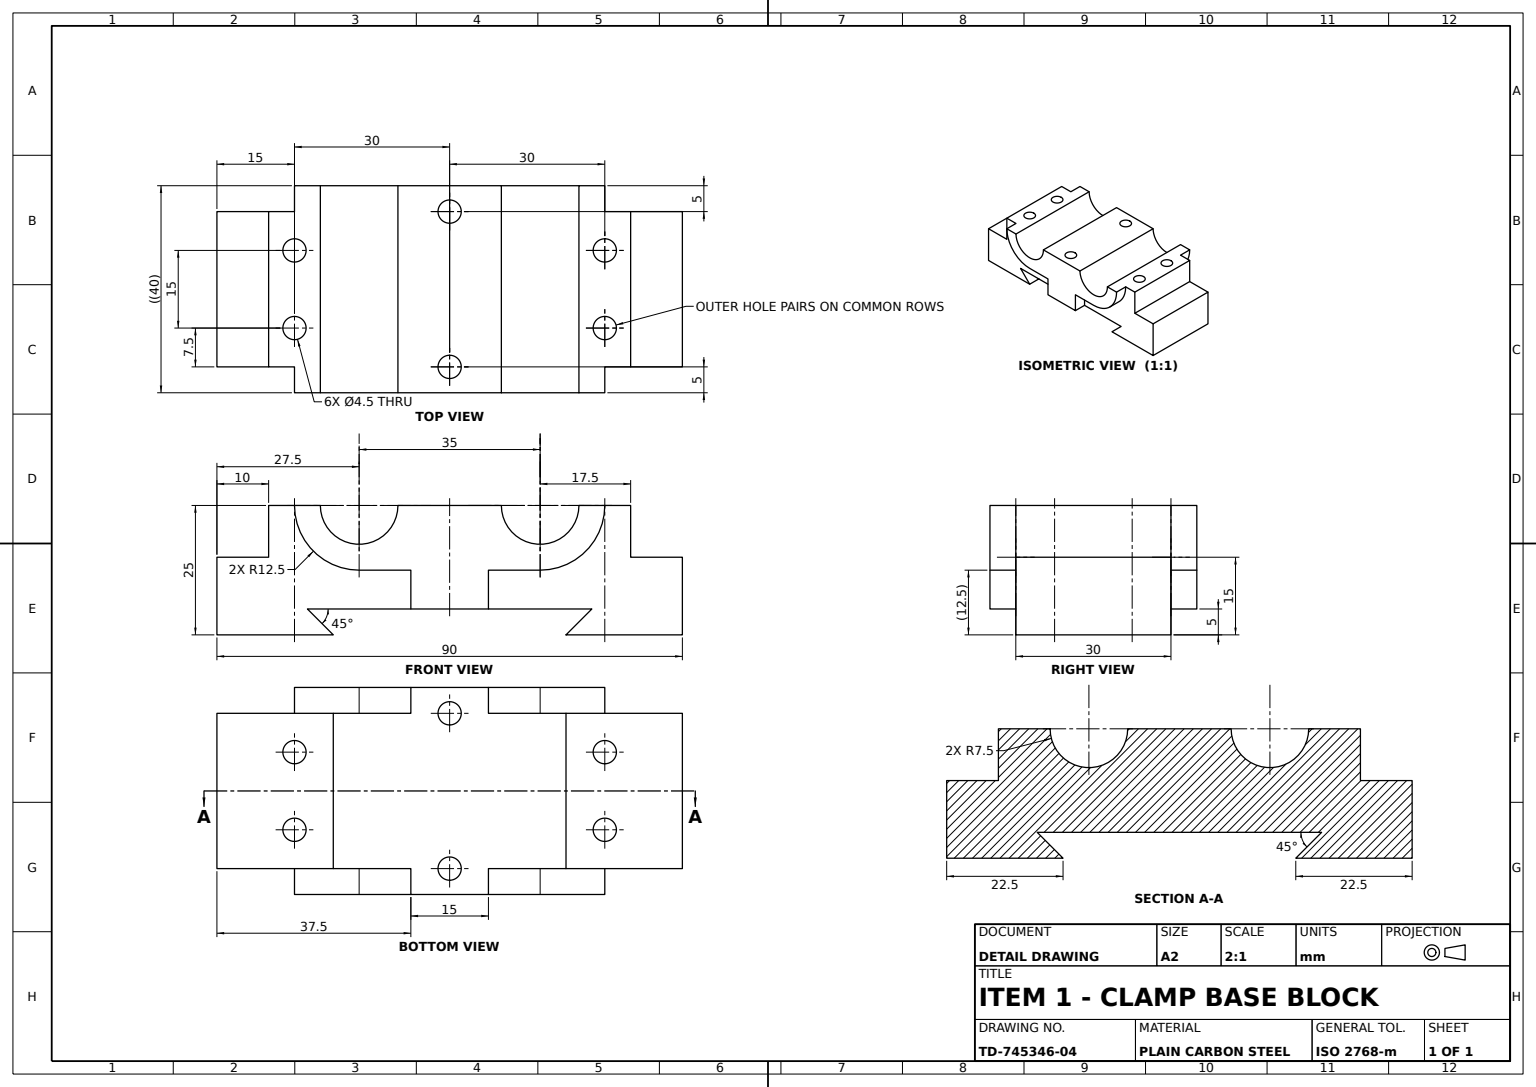
ISO-10303-21;
HEADER;
FILE_DESCRIPTION((''),'2;1');
FILE_NAME('','',(''),(''),'','','');
FILE_SCHEMA(('AUTOMOTIVE_DESIGN'));
ENDSEC;
DATA;
#1=APPLICATION_CONTEXT('');
#2=PRODUCT_CONTEXT('',#1,'mechanical');
#3=PRODUCT('','','',(#2));
#4=PRODUCT_DEFINITION_FORMATION('','',#3);
#5=PRODUCT_DEFINITION_CONTEXT('',#1,'design');
#6=PRODUCT_DEFINITION('','',#4,#5);
#7=PRODUCT_DEFINITION_SHAPE('','',#6);
#8=(LENGTH_UNIT()NAMED_UNIT(*)SI_UNIT(.MILLI.,.METRE.));
#9=(NAMED_UNIT(*)PLANE_ANGLE_UNIT()SI_UNIT($,.RADIAN.));
#10=(NAMED_UNIT(*)SI_UNIT($,.STERADIAN.)SOLID_ANGLE_UNIT());
#11=UNCERTAINTY_MEASURE_WITH_UNIT(LENGTH_MEASURE(1.E-05),#8,'distance_accuracy_value','');
#12=(GEOMETRIC_REPRESENTATION_CONTEXT(3)GLOBAL_UNCERTAINTY_ASSIGNED_CONTEXT((#11))GLOBAL_UNIT_ASSIGNED_CONTEXT((#8,#9,#10))REPRESENTATION_CONTEXT('',''));
#13=CARTESIAN_POINT('',(-25.,18.587361,-20.));
#14=VERTEX_POINT('',#13);
#15=CARTESIAN_POINT('',(-30.,18.587361,-20.));
#16=VERTEX_POINT('',#15);
#17=CARTESIAN_POINT('',(-35.,18.587361,-20.));
#18=DIRECTION('',(-1.,0.,0.));
#19=VECTOR('',#18,1000.);
#20=LINE('',#17,#19);
#21=EDGE_CURVE('',#14,#16,#20,.T.);
#22=ORIENTED_EDGE('',*,*,#21,.F.);
#23=CARTESIAN_POINT('',(-10.,18.587361,-20.));
#24=VERTEX_POINT('',#23);
#25=CARTESIAN_POINT('',(-17.5,18.587361,-20.));
#26=DIRECTION('',(0.,0.,1.));
#27=DIRECTION('',(1.,0.,0.));
#28=AXIS2_PLACEMENT_3D('',#25,#26,#27);
#29=CIRCLE('',#28,7.5);
#30=EDGE_CURVE('',#14,#24,#29,.T.);
#31=ORIENTED_EDGE('',*,*,#30,.T.);
#32=CARTESIAN_POINT('',(10.,18.587361,-20.));
#33=VERTEX_POINT('',#32);
#34=EDGE_CURVE('',#33,#24,#20,.T.);
#35=ORIENTED_EDGE('',*,*,#34,.F.);
#36=CARTESIAN_POINT('',(25.,18.587361,-20.));
#37=VERTEX_POINT('',#36);
#38=CARTESIAN_POINT('',(17.5,18.587361,-20.));
#39=DIRECTION('',(0.,0.,-1.));
#40=AXIS2_PLACEMENT_3D('',#38,#39,#27);
#41=CIRCLE('',#40,7.5);
#42=EDGE_CURVE('',#37,#33,#41,.T.);
#43=ORIENTED_EDGE('',*,*,#42,.F.);
#44=CARTESIAN_POINT('',(30.,18.587361,-20.));
#45=VERTEX_POINT('',#44);
#46=EDGE_CURVE('',#45,#37,#20,.T.);
#47=ORIENTED_EDGE('',*,*,#46,.F.);
#48=CARTESIAN_POINT('',(17.5,6.087361,-20.));
#49=VERTEX_POINT('',#48);
#50=CIRCLE('',#40,12.5);
#51=EDGE_CURVE('',#45,#49,#50,.T.);
#52=ORIENTED_EDGE('',*,*,#51,.T.);
#53=CARTESIAN_POINT('',(7.5,6.087361,-20.));
#54=VERTEX_POINT('',#53);
#55=CARTESIAN_POINT('',(0.,6.087361,-20.));
#56=VECTOR('',#27,1000.);
#57=LINE('',#55,#56);
#58=EDGE_CURVE('',#54,#49,#57,.T.);
#59=ORIENTED_EDGE('',*,*,#58,.F.);
#60=CARTESIAN_POINT('',(7.5,-1.412639,-20.));
#61=VERTEX_POINT('',#60);
#62=CARTESIAN_POINT('',(7.5,0.,-20.));
#63=DIRECTION('',(0.,1.,0.));
#64=VECTOR('',#63,1000.);
#65=LINE('',#62,#64);
#66=EDGE_CURVE('',#61,#54,#65,.T.);
#67=ORIENTED_EDGE('',*,*,#66,.F.);
#68=CARTESIAN_POINT('',(-7.5,-1.412639,-20.));
#69=VERTEX_POINT('',#68);
#70=CARTESIAN_POINT('',(-27.5,-1.412639,-20.));
#71=LINE('',#70,#56);
#72=EDGE_CURVE('',#69,#61,#71,.T.);
#73=ORIENTED_EDGE('',*,*,#72,.F.);
#74=CARTESIAN_POINT('',(-7.5,6.087361,-20.));
#75=VERTEX_POINT('',#74);
#76=CARTESIAN_POINT('',(-7.5,0.,-20.));
#77=LINE('',#76,#64);
#78=EDGE_CURVE('',#69,#75,#77,.T.);
#79=ORIENTED_EDGE('',*,*,#78,.T.);
#80=CARTESIAN_POINT('',(-17.5,6.087361,-20.));
#81=VERTEX_POINT('',#80);
#82=LINE('',#55,#19);
#83=EDGE_CURVE('',#75,#81,#82,.T.);
#84=ORIENTED_EDGE('',*,*,#83,.T.);
#85=CIRCLE('',#28,12.5);
#86=EDGE_CURVE('',#16,#81,#85,.T.);
#87=ORIENTED_EDGE('',*,*,#86,.F.);
#88=EDGE_LOOP('',(#22,#31,#35,#43,#47,#52,#59,#67,#73,#79,#84,#87));
#89=FACE_OUTER_BOUND('',#88,.T.);
#90=CARTESIAN_POINT('',(0.,0.,-20.));
#91=AXIS2_PLACEMENT_3D('',#90,#26,#27);
#92=PLANE('',#91);
#93=ADVANCED_FACE('',(#89),#92,.F.);
#94=CARTESIAN_POINT('',(35.,8.587361,15.));
#95=VERTEX_POINT('',#94);
#96=CARTESIAN_POINT('',(35.,8.587361,-15.));
#97=VERTEX_POINT('',#96);
#98=CARTESIAN_POINT('',(35.,8.587361,20.));
#99=VECTOR('',#39,1000.);
#100=LINE('',#98,#99);
#101=EDGE_CURVE('',#95,#97,#100,.T.);
#102=ORIENTED_EDGE('',*,*,#101,.T.);
#103=CARTESIAN_POINT('',(35.,18.587361,-15.));
#104=VERTEX_POINT('',#103);
#105=DIRECTION('',(0.,-1.,0.));
#106=VECTOR('',#105,1000.);
#107=LINE('',#103,#106);
#108=EDGE_CURVE('',#104,#97,#107,.T.);
#109=ORIENTED_EDGE('',*,*,#108,.F.);
#110=CARTESIAN_POINT('',(35.,18.587361,15.));
#111=VERTEX_POINT('',#110);
#112=CARTESIAN_POINT('',(35.,18.587361,20.));
#113=LINE('',#112,#99);
#114=EDGE_CURVE('',#111,#104,#113,.T.);
#115=ORIENTED_EDGE('',*,*,#114,.F.);
#116=LINE('',#110,#64);
#117=EDGE_CURVE('',#95,#111,#116,.T.);
#118=ORIENTED_EDGE('',*,*,#117,.F.);
#119=EDGE_LOOP('',(#102,#109,#115,#118));
#120=FACE_OUTER_BOUND('',#119,.T.);
#121=AXIS2_PLACEMENT_3D('',#112,#18,#26);
#122=PLANE('',#121);
#123=ADVANCED_FACE('',(#120),#122,.F.);
#124=CARTESIAN_POINT('',(30.,-6.412639,9.75));
#125=VERTEX_POINT('',#124);
#126=CARTESIAN_POINT('',(30.,18.587361,9.75));
#127=VERTEX_POINT('',#126);
#128=CARTESIAN_POINT('',(30.,-21.412639,9.75));
#129=LINE('',#128,#64);
#130=EDGE_CURVE('',#125,#127,#129,.T.);
#131=ORIENTED_EDGE('',*,*,#130,.F.);
#132=CARTESIAN_POINT('',(30.,-6.412639,5.25));
#133=VERTEX_POINT('',#132);
#134=CARTESIAN_POINT('',(30.,-6.412639,7.5));
#135=AXIS2_PLACEMENT_3D('',#134,#63,#18);
#136=CIRCLE('',#135,2.25);
#137=EDGE_CURVE('',#133,#125,#136,.T.);
#138=ORIENTED_EDGE('',*,*,#137,.F.);
#139=CARTESIAN_POINT('',(30.,18.587361,5.25));
#140=VERTEX_POINT('',#139);
#141=CARTESIAN_POINT('',(30.,-21.412639,5.25));
#142=LINE('',#141,#64);
#143=EDGE_CURVE('',#133,#140,#142,.T.);
#144=ORIENTED_EDGE('',*,*,#143,.T.);
#145=CARTESIAN_POINT('',(30.,18.587361,7.5));
#146=AXIS2_PLACEMENT_3D('',#145,#63,#26);
#147=CIRCLE('',#146,2.25);
#148=EDGE_CURVE('',#140,#127,#147,.T.);
#149=ORIENTED_EDGE('',*,*,#148,.T.);
#150=EDGE_LOOP('',(#131,#138,#144,#149));
#151=FACE_OUTER_BOUND('',#150,.T.);
#152=CARTESIAN_POINT('',(30.,-21.412639,7.5));
#153=AXIS2_PLACEMENT_3D('',#152,#63,#26);
#154=CYLINDRICAL_SURFACE('',#153,2.25);
#155=ADVANCED_FACE('',(#151),#154,.F.);
#156=CARTESIAN_POINT('',(-7.5,-1.412639,-15.));
#157=VERTEX_POINT('',#156);
#158=CARTESIAN_POINT('',(-7.5,6.087361,-15.));
#159=VERTEX_POINT('',#158);
#160=CARTESIAN_POINT('',(-7.5,0.,-15.));
#161=LINE('',#160,#64);
#162=EDGE_CURVE('',#157,#159,#161,.T.);
#163=ORIENTED_EDGE('',*,*,#162,.T.);
#164=CARTESIAN_POINT('',(-7.5,6.087361,-125.));
#165=VECTOR('',#26,1000.);
#166=LINE('',#164,#165);
#167=EDGE_CURVE('',#75,#159,#166,.T.);
#168=ORIENTED_EDGE('',*,*,#167,.F.);
#169=ORIENTED_EDGE('',*,*,#78,.F.);
#170=CARTESIAN_POINT('',(-7.5,-1.412639,-125.));
#171=LINE('',#170,#165);
#172=EDGE_CURVE('',#69,#157,#171,.T.);
#173=ORIENTED_EDGE('',*,*,#172,.T.);
#174=EDGE_LOOP('',(#163,#168,#169,#173));
#175=FACE_OUTER_BOUND('',#174,.T.);
#176=CARTESIAN_POINT('',(-7.5,0.,-125.));
#177=AXIS2_PLACEMENT_3D('',#176,#27,#39);
#178=PLANE('',#177);
#179=ADVANCED_FACE('',(#175),#178,.F.);
#180=EDGE_CURVE('',#125,#133,#136,.T.);
#181=ORIENTED_EDGE('',*,*,#180,.F.);
#182=ORIENTED_EDGE('',*,*,#130,.T.);
#183=EDGE_CURVE('',#127,#140,#147,.T.);
#184=ORIENTED_EDGE('',*,*,#183,.T.);
#185=ORIENTED_EDGE('',*,*,#143,.F.);
#186=EDGE_LOOP('',(#181,#182,#184,#185));
#187=FACE_OUTER_BOUND('',#186,.T.);
#188=ADVANCED_FACE('',(#187),#154,.F.);
#189=CARTESIAN_POINT('',(0.,18.587361,-17.25));
#190=VERTEX_POINT('',#189);
#191=CARTESIAN_POINT('',(0.,18.587361,-12.75));
#192=VERTEX_POINT('',#191);
#193=CARTESIAN_POINT('',(0.,18.587361,-15.));
#194=AXIS2_PLACEMENT_3D('',#193,#63,#26);
#195=CIRCLE('',#194,2.25);
#196=EDGE_CURVE('',#190,#192,#195,.T.);
#197=ORIENTED_EDGE('',*,*,#196,.T.);
#198=CARTESIAN_POINT('',(0.,-1.412639,-12.75));
#199=VERTEX_POINT('',#198);
#200=CARTESIAN_POINT('',(0.,-21.412639,-12.75));
#201=LINE('',#200,#64);
#202=EDGE_CURVE('',#199,#192,#201,.T.);
#203=ORIENTED_EDGE('',*,*,#202,.F.);
#204=CARTESIAN_POINT('',(0.,-1.412639,-17.25));
#205=VERTEX_POINT('',#204);
#206=CARTESIAN_POINT('',(0.,-1.412639,-15.));
#207=AXIS2_PLACEMENT_3D('',#206,#63,#18);
#208=CIRCLE('',#207,2.25);
#209=EDGE_CURVE('',#205,#199,#208,.T.);
#210=ORIENTED_EDGE('',*,*,#209,.F.);
#211=CARTESIAN_POINT('',(0.,-21.412639,-17.25));
#212=LINE('',#211,#64);
#213=EDGE_CURVE('',#205,#190,#212,.T.);
#214=ORIENTED_EDGE('',*,*,#213,.T.);
#215=EDGE_LOOP('',(#197,#203,#210,#214));
#216=FACE_OUTER_BOUND('',#215,.T.);
#217=CARTESIAN_POINT('',(0.,-21.412639,-15.));
#218=AXIS2_PLACEMENT_3D('',#217,#63,#26);
#219=CYLINDRICAL_SURFACE('',#218,2.25);
#220=ADVANCED_FACE('',(#216),#219,.F.);
#221=CARTESIAN_POINT('',(-30.,-6.412639,5.25));
#222=VERTEX_POINT('',#221);
#223=CARTESIAN_POINT('',(-30.,18.587361,5.25));
#224=VERTEX_POINT('',#223);
#225=CARTESIAN_POINT('',(-30.,-21.412639,5.25));
#226=LINE('',#225,#64);
#227=EDGE_CURVE('',#222,#224,#226,.T.);
#228=ORIENTED_EDGE('',*,*,#227,.T.);
#229=CARTESIAN_POINT('',(-30.,18.587361,9.75));
#230=VERTEX_POINT('',#229);
#231=CARTESIAN_POINT('',(-30.,18.587361,7.5));
#232=AXIS2_PLACEMENT_3D('',#231,#63,#39);
#233=CIRCLE('',#232,2.25);
#234=EDGE_CURVE('',#224,#230,#233,.T.);
#235=ORIENTED_EDGE('',*,*,#234,.T.);
#236=CARTESIAN_POINT('',(-30.,-6.412639,9.75));
#237=VERTEX_POINT('',#236);
#238=CARTESIAN_POINT('',(-30.,-21.412639,9.75));
#239=LINE('',#238,#64);
#240=EDGE_CURVE('',#237,#230,#239,.T.);
#241=ORIENTED_EDGE('',*,*,#240,.F.);
#242=CARTESIAN_POINT('',(-30.,-6.412639,7.5));
#243=AXIS2_PLACEMENT_3D('',#242,#63,#18);
#244=CIRCLE('',#243,2.25);
#245=EDGE_CURVE('',#222,#237,#244,.T.);
#246=ORIENTED_EDGE('',*,*,#245,.F.);
#247=EDGE_LOOP('',(#228,#235,#241,#246));
#248=FACE_OUTER_BOUND('',#247,.T.);
#249=CARTESIAN_POINT('',(-30.,-21.412639,7.5));
#250=AXIS2_PLACEMENT_3D('',#249,#63,#26);
#251=CYLINDRICAL_SURFACE('',#250,2.25);
#252=ADVANCED_FACE('',(#248),#251,.F.);
#253=CARTESIAN_POINT('',(-30.,18.587361,-9.75));
#254=VERTEX_POINT('',#253);
#255=CARTESIAN_POINT('',(-30.,18.587361,-5.25));
#256=VERTEX_POINT('',#255);
#257=CARTESIAN_POINT('',(-30.,18.587361,-7.5));
#258=AXIS2_PLACEMENT_3D('',#257,#63,#26);
#259=CIRCLE('',#258,2.25);
#260=EDGE_CURVE('',#254,#256,#259,.T.);
#261=ORIENTED_EDGE('',*,*,#260,.T.);
#262=CARTESIAN_POINT('',(-30.,-6.412639,-5.25));
#263=VERTEX_POINT('',#262);
#264=CARTESIAN_POINT('',(-30.,-21.412639,-5.25));
#265=LINE('',#264,#64);
#266=EDGE_CURVE('',#263,#256,#265,.T.);
#267=ORIENTED_EDGE('',*,*,#266,.F.);
#268=CARTESIAN_POINT('',(-30.,-6.412639,-9.75));
#269=VERTEX_POINT('',#268);
#270=CARTESIAN_POINT('',(-30.,-6.412639,-7.5));
#271=AXIS2_PLACEMENT_3D('',#270,#63,#18);
#272=CIRCLE('',#271,2.25);
#273=EDGE_CURVE('',#269,#263,#272,.T.);
#274=ORIENTED_EDGE('',*,*,#273,.F.);
#275=CARTESIAN_POINT('',(-30.,-21.412639,-9.75));
#276=LINE('',#275,#64);
#277=EDGE_CURVE('',#269,#254,#276,.T.);
#278=ORIENTED_EDGE('',*,*,#277,.T.);
#279=EDGE_LOOP('',(#261,#267,#274,#278));
#280=FACE_OUTER_BOUND('',#279,.T.);
#281=CARTESIAN_POINT('',(-30.,-21.412639,-7.5));
#282=AXIS2_PLACEMENT_3D('',#281,#63,#26);
#283=CYLINDRICAL_SURFACE('',#282,2.25);
#284=ADVANCED_FACE('',(#280),#283,.F.);
#285=CARTESIAN_POINT('',(-30.,18.587361,-15.));
#286=VERTEX_POINT('',#285);
#287=CARTESIAN_POINT('',(-35.,18.587361,-15.));
#288=VERTEX_POINT('',#287);
#289=LINE('',#285,#19);
#290=EDGE_CURVE('',#286,#288,#289,.T.);
#291=ORIENTED_EDGE('',*,*,#290,.F.);
#292=CARTESIAN_POINT('',(-17.5,6.087361,-15.));
#293=VERTEX_POINT('',#292);
#294=CARTESIAN_POINT('',(-17.5,18.587361,-15.));
#295=AXIS2_PLACEMENT_3D('',#294,#26,#27);
#296=CIRCLE('',#295,12.5);
#297=EDGE_CURVE('',#286,#293,#296,.T.);
#298=ORIENTED_EDGE('',*,*,#297,.T.);
#299=CARTESIAN_POINT('',(0.,6.087361,-15.));
#300=LINE('',#299,#19);
#301=EDGE_CURVE('',#159,#293,#300,.T.);
#302=ORIENTED_EDGE('',*,*,#301,.F.);
#303=ORIENTED_EDGE('',*,*,#162,.F.);
#304=CARTESIAN_POINT('',(-27.5,-1.412639,-15.));
#305=VERTEX_POINT('',#304);
#306=LINE('',#206,#19);
#307=EDGE_CURVE('',#157,#305,#306,.T.);
#308=ORIENTED_EDGE('',*,*,#307,.T.);
#309=CARTESIAN_POINT('',(-22.5,-6.412639,-15.));
#310=VERTEX_POINT('',#309);
#311=CARTESIAN_POINT('',(-14.45632,-14.45632,-15.));
#312=DIRECTION('',(0.707106781,-0.707106781,0.));
#313=VECTOR('',#312,1000.);
#314=LINE('',#311,#313);
#315=EDGE_CURVE('',#305,#310,#314,.T.);
#316=ORIENTED_EDGE('',*,*,#315,.T.);
#317=CARTESIAN_POINT('',(-45.,-6.412639,-15.));
#318=VERTEX_POINT('',#317);
#319=LINE('',#317,#19);
#320=EDGE_CURVE('',#310,#318,#319,.T.);
#321=ORIENTED_EDGE('',*,*,#320,.T.);
#322=CARTESIAN_POINT('',(-45.,8.587361,-15.));
#323=VERTEX_POINT('',#322);
#324=CARTESIAN_POINT('',(-45.,-21.412639,-15.));
#325=LINE('',#324,#64);
#326=EDGE_CURVE('',#318,#323,#325,.T.);
#327=ORIENTED_EDGE('',*,*,#326,.T.);
#328=CARTESIAN_POINT('',(-35.,8.587361,-15.));
#329=VERTEX_POINT('',#328);
#330=LINE('',#328,#56);
#331=EDGE_CURVE('',#323,#329,#330,.T.);
#332=ORIENTED_EDGE('',*,*,#331,.T.);
#333=LINE('',#287,#64);
#334=EDGE_CURVE('',#329,#288,#333,.T.);
#335=ORIENTED_EDGE('',*,*,#334,.T.);
#336=EDGE_LOOP('',(#291,#298,#302,#303,#308,#316,#321,#327,#332,#335));
#337=FACE_OUTER_BOUND('',#336,.T.);
#338=CARTESIAN_POINT('',(-30.,-21.412639,-15.));
#339=AXIS2_PLACEMENT_3D('',#338,#39,#18);
#340=PLANE('',#339);
#341=ADVANCED_FACE('',(#337),#340,.T.);
#342=ORIENTED_EDGE('',*,*,#326,.F.);
#343=CARTESIAN_POINT('',(-45.,-6.412639,15.));
#344=VERTEX_POINT('',#343);
#345=CARTESIAN_POINT('',(-45.,-6.412639,20.));
#346=LINE('',#345,#99);
#347=EDGE_CURVE('',#344,#318,#346,.T.);
#348=ORIENTED_EDGE('',*,*,#347,.F.);
#349=CARTESIAN_POINT('',(-45.,8.587361,15.));
#350=VERTEX_POINT('',#349);
#351=CARTESIAN_POINT('',(-45.,-21.412639,15.));
#352=LINE('',#351,#64);
#353=EDGE_CURVE('',#344,#350,#352,.T.);
#354=ORIENTED_EDGE('',*,*,#353,.T.);
#355=CARTESIAN_POINT('',(-45.,8.587361,20.));
#356=LINE('',#355,#99);
#357=EDGE_CURVE('',#350,#323,#356,.T.);
#358=ORIENTED_EDGE('',*,*,#357,.T.);
#359=EDGE_LOOP('',(#342,#348,#354,#358));
#360=FACE_OUTER_BOUND('',#359,.T.);
#361=AXIS2_PLACEMENT_3D('',#355,#27,#39);
#362=PLANE('',#361);
#363=ADVANCED_FACE('',(#360),#362,.F.);
#364=CARTESIAN_POINT('',(30.,18.587361,15.));
#365=VERTEX_POINT('',#364);
#366=CARTESIAN_POINT('',(17.5,6.087361,15.));
#367=VERTEX_POINT('',#366);
#368=CARTESIAN_POINT('',(17.5,18.587361,15.));
#369=AXIS2_PLACEMENT_3D('',#368,#39,#18);
#370=CIRCLE('',#369,12.5);
#371=EDGE_CURVE('',#365,#367,#370,.T.);
#372=ORIENTED_EDGE('',*,*,#371,.T.);
#373=CARTESIAN_POINT('',(7.5,6.087361,15.));
#374=VERTEX_POINT('',#373);
#375=CARTESIAN_POINT('',(0.,6.087361,15.));
#376=LINE('',#375,#56);
#377=EDGE_CURVE('',#374,#367,#376,.T.);
#378=ORIENTED_EDGE('',*,*,#377,.F.);
#379=CARTESIAN_POINT('',(7.5,-1.412639,15.));
#380=VERTEX_POINT('',#379);
#381=CARTESIAN_POINT('',(7.5,0.,15.));
#382=LINE('',#381,#64);
#383=EDGE_CURVE('',#380,#374,#382,.T.);
#384=ORIENTED_EDGE('',*,*,#383,.F.);
#385=CARTESIAN_POINT('',(27.5,-1.412639,15.));
#386=VERTEX_POINT('',#385);
#387=CARTESIAN_POINT('',(0.,-1.412639,15.));
#388=LINE('',#387,#56);
#389=EDGE_CURVE('',#380,#386,#388,.T.);
#390=ORIENTED_EDGE('',*,*,#389,.T.);
#391=CARTESIAN_POINT('',(22.5,-6.412639,15.));
#392=VERTEX_POINT('',#391);
#393=CARTESIAN_POINT('',(14.45632,-14.45632,15.));
#394=DIRECTION('',(-0.707106781,-0.707106781,0.));
#395=VECTOR('',#394,1000.);
#396=LINE('',#393,#395);
#397=EDGE_CURVE('',#386,#392,#396,.T.);
#398=ORIENTED_EDGE('',*,*,#397,.T.);
#399=CARTESIAN_POINT('',(45.,-6.412639,15.));
#400=VERTEX_POINT('',#399);
#401=LINE('',#399,#56);
#402=EDGE_CURVE('',#392,#400,#401,.T.);
#403=ORIENTED_EDGE('',*,*,#402,.T.);
#404=CARTESIAN_POINT('',(45.,8.587361,15.));
#405=VERTEX_POINT('',#404);
#406=CARTESIAN_POINT('',(45.,-21.412639,15.));
#407=LINE('',#406,#64);
#408=EDGE_CURVE('',#400,#405,#407,.T.);
#409=ORIENTED_EDGE('',*,*,#408,.T.);
#410=LINE('',#94,#19);
#411=EDGE_CURVE('',#405,#95,#410,.T.);
#412=ORIENTED_EDGE('',*,*,#411,.T.);
#413=ORIENTED_EDGE('',*,*,#117,.T.);
#414=CARTESIAN_POINT('',(45.,18.587361,15.));
#415=LINE('',#414,#56);
#416=EDGE_CURVE('',#365,#111,#415,.T.);
#417=ORIENTED_EDGE('',*,*,#416,.F.);
#418=EDGE_LOOP('',(#372,#378,#384,#390,#398,#403,#409,#412,#413,#417));
#419=FACE_OUTER_BOUND('',#418,.T.);
#420=AXIS2_PLACEMENT_3D('',#406,#26,#27);
#421=PLANE('',#420);
#422=ADVANCED_FACE('',(#419),#421,.T.);
#423=ORIENTED_EDGE('',*,*,#213,.F.);
#424=EDGE_CURVE('',#199,#205,#208,.T.);
#425=ORIENTED_EDGE('',*,*,#424,.F.);
#426=ORIENTED_EDGE('',*,*,#202,.T.);
#427=EDGE_CURVE('',#192,#190,#195,.T.);
#428=ORIENTED_EDGE('',*,*,#427,.T.);
#429=EDGE_LOOP('',(#423,#425,#426,#428));
#430=FACE_OUTER_BOUND('',#429,.T.);
#431=ADVANCED_FACE('',(#430),#219,.F.);
#432=CARTESIAN_POINT('',(-17.5,6.087361,-125.));
#433=LINE('',#432,#165);
#434=EDGE_CURVE('',#81,#293,#433,.T.);
#435=ORIENTED_EDGE('',*,*,#434,.F.);
#436=ORIENTED_EDGE('',*,*,#83,.F.);
#437=ORIENTED_EDGE('',*,*,#167,.T.);
#438=ORIENTED_EDGE('',*,*,#301,.T.);
#439=EDGE_LOOP('',(#435,#436,#437,#438));
#440=FACE_OUTER_BOUND('',#439,.T.);
#441=CARTESIAN_POINT('',(0.,6.087361,-125.));
#442=AXIS2_PLACEMENT_3D('',#441,#63,#18);
#443=PLANE('',#442);
#444=ADVANCED_FACE('',(#440),#443,.F.);
#445=ORIENTED_EDGE('',*,*,#34,.T.);
#446=CARTESIAN_POINT('',(-10.,18.587361,20.));
#447=VERTEX_POINT('',#446);
#448=CARTESIAN_POINT('',(-10.,18.587361,-40.));
#449=LINE('',#448,#165);
#450=EDGE_CURVE('',#24,#447,#449,.T.);
#451=ORIENTED_EDGE('',*,*,#450,.T.);
#452=CARTESIAN_POINT('',(10.,18.587361,20.));
#453=VERTEX_POINT('',#452);
#454=LINE('',#112,#19);
#455=EDGE_CURVE('',#453,#447,#454,.T.);
#456=ORIENTED_EDGE('',*,*,#455,.F.);
#457=CARTESIAN_POINT('',(10.,18.587361,-40.));
#458=LINE('',#457,#165);
#459=EDGE_CURVE('',#33,#453,#458,.T.);
#460=ORIENTED_EDGE('',*,*,#459,.F.);
#461=EDGE_LOOP('',(#445,#451,#456,#460));
#462=FACE_OUTER_BOUND('',#461,.T.);
#463=ORIENTED_EDGE('',*,*,#427,.F.);
#464=ORIENTED_EDGE('',*,*,#196,.F.);
#465=EDGE_LOOP('',(#463,#464));
#466=FACE_BOUND('',#465,.T.);
#467=CARTESIAN_POINT('',(0.,18.587361,17.25));
#468=VERTEX_POINT('',#467);
#469=CARTESIAN_POINT('',(0.,18.587361,12.75));
#470=VERTEX_POINT('',#469);
#471=CARTESIAN_POINT('',(0.,18.587361,15.));
#472=AXIS2_PLACEMENT_3D('',#471,#63,#39);
#473=CIRCLE('',#472,2.25);
#474=EDGE_CURVE('',#468,#470,#473,.T.);
#475=ORIENTED_EDGE('',*,*,#474,.F.);
#476=EDGE_CURVE('',#470,#468,#473,.T.);
#477=ORIENTED_EDGE('',*,*,#476,.F.);
#478=EDGE_LOOP('',(#475,#477));
#479=FACE_BOUND('',#478,.T.);
#480=CARTESIAN_POINT('',(-35.,18.587361,20.));
#481=AXIS2_PLACEMENT_3D('',#480,#105,#39);
#482=PLANE('',#481);
#483=ADVANCED_FACE('',(#462,#466,#479),#482,.F.);
#484=CARTESIAN_POINT('',(-7.5,-1.412639,15.));
#485=VERTEX_POINT('',#484);
#486=CARTESIAN_POINT('',(-7.5,-1.412639,20.));
#487=VERTEX_POINT('',#486);
#488=LINE('',#486,#165);
#489=EDGE_CURVE('',#485,#487,#488,.T.);
#490=ORIENTED_EDGE('',*,*,#489,.T.);
#491=CARTESIAN_POINT('',(-7.5,6.087361,20.));
#492=VERTEX_POINT('',#491);
#493=CARTESIAN_POINT('',(-7.5,0.,20.));
#494=LINE('',#493,#106);
#495=EDGE_CURVE('',#492,#487,#494,.T.);
#496=ORIENTED_EDGE('',*,*,#495,.F.);
#497=CARTESIAN_POINT('',(-7.5,6.087361,15.));
#498=VERTEX_POINT('',#497);
#499=CARTESIAN_POINT('',(-7.5,6.087361,125.));
#500=LINE('',#499,#99);
#501=EDGE_CURVE('',#492,#498,#500,.T.);
#502=ORIENTED_EDGE('',*,*,#501,.T.);
#503=CARTESIAN_POINT('',(-7.5,0.,15.));
#504=LINE('',#503,#64);
#505=EDGE_CURVE('',#485,#498,#504,.T.);
#506=ORIENTED_EDGE('',*,*,#505,.F.);
#507=EDGE_LOOP('',(#490,#496,#502,#506));
#508=FACE_OUTER_BOUND('',#507,.T.);
#509=CARTESIAN_POINT('',(-7.5,0.,125.));
#510=AXIS2_PLACEMENT_3D('',#509,#18,#26);
#511=PLANE('',#510);
#512=ADVANCED_FACE('',(#508),#511,.T.);
#513=CARTESIAN_POINT('',(0.,-1.412639,17.25));
#514=VERTEX_POINT('',#513);
#515=CARTESIAN_POINT('',(0.,-1.412639,12.75));
#516=VERTEX_POINT('',#515);
#517=AXIS2_PLACEMENT_3D('',#387,#63,#18);
#518=CIRCLE('',#517,2.25);
#519=EDGE_CURVE('',#514,#516,#518,.T.);
#520=ORIENTED_EDGE('',*,*,#519,.F.);
#521=CARTESIAN_POINT('',(0.,-21.412639,17.25));
#522=LINE('',#521,#64);
#523=EDGE_CURVE('',#514,#468,#522,.T.);
#524=ORIENTED_EDGE('',*,*,#523,.T.);
#525=ORIENTED_EDGE('',*,*,#474,.T.);
#526=CARTESIAN_POINT('',(0.,-21.412639,12.75));
#527=LINE('',#526,#64);
#528=EDGE_CURVE('',#516,#470,#527,.T.);
#529=ORIENTED_EDGE('',*,*,#528,.F.);
#530=EDGE_LOOP('',(#520,#524,#525,#529));
#531=FACE_OUTER_BOUND('',#530,.T.);
#532=CARTESIAN_POINT('',(0.,-21.412639,15.));
#533=AXIS2_PLACEMENT_3D('',#532,#63,#26);
#534=CYLINDRICAL_SURFACE('',#533,2.25);
#535=ADVANCED_FACE('',(#531),#534,.F.);
#536=ORIENTED_EDGE('',*,*,#408,.F.);
#537=CARTESIAN_POINT('',(45.,-6.412639,-15.));
#538=VERTEX_POINT('',#537);
#539=CARTESIAN_POINT('',(45.,-6.412639,20.));
#540=LINE('',#539,#99);
#541=EDGE_CURVE('',#400,#538,#540,.T.);
#542=ORIENTED_EDGE('',*,*,#541,.T.);
#543=CARTESIAN_POINT('',(45.,8.587361,-15.));
#544=VERTEX_POINT('',#543);
#545=CARTESIAN_POINT('',(45.,-21.412639,-15.));
#546=LINE('',#545,#64);
#547=EDGE_CURVE('',#538,#544,#546,.T.);
#548=ORIENTED_EDGE('',*,*,#547,.T.);
#549=CARTESIAN_POINT('',(45.,8.587361,20.));
#550=LINE('',#549,#99);
#551=EDGE_CURVE('',#405,#544,#550,.T.);
#552=ORIENTED_EDGE('',*,*,#551,.F.);
#553=EDGE_LOOP('',(#536,#542,#548,#552));
#554=FACE_OUTER_BOUND('',#553,.T.);
#555=AXIS2_PLACEMENT_3D('',#549,#18,#26);
#556=PLANE('',#555);
#557=ADVANCED_FACE('',(#554),#556,.F.);
#558=ORIENTED_EDGE('',*,*,#501,.F.);
#559=CARTESIAN_POINT('',(-17.5,6.087361,20.));
#560=VERTEX_POINT('',#559);
#561=CARTESIAN_POINT('',(0.,6.087361,20.));
#562=LINE('',#561,#56);
#563=EDGE_CURVE('',#560,#492,#562,.T.);
#564=ORIENTED_EDGE('',*,*,#563,.F.);
#565=CARTESIAN_POINT('',(-17.5,6.087361,15.));
#566=VERTEX_POINT('',#565);
#567=CARTESIAN_POINT('',(-17.5,6.087361,125.));
#568=LINE('',#567,#99);
#569=EDGE_CURVE('',#560,#566,#568,.T.);
#570=ORIENTED_EDGE('',*,*,#569,.T.);
#571=LINE('',#375,#19);
#572=EDGE_CURVE('',#498,#566,#571,.T.);
#573=ORIENTED_EDGE('',*,*,#572,.F.);
#574=EDGE_LOOP('',(#558,#564,#570,#573));
#575=FACE_OUTER_BOUND('',#574,.T.);
#576=CARTESIAN_POINT('',(0.,6.087361,125.));
#577=AXIS2_PLACEMENT_3D('',#576,#105,#27);
#578=PLANE('',#577);
#579=ADVANCED_FACE('',(#575),#578,.T.);
#580=CARTESIAN_POINT('',(22.5,-6.412639,-15.));
#581=VERTEX_POINT('',#580);
#582=LINE('',#537,#19);
#583=EDGE_CURVE('',#538,#581,#582,.T.);
#584=ORIENTED_EDGE('',*,*,#583,.T.);
#585=CARTESIAN_POINT('',(27.5,-1.412639,-15.));
#586=VERTEX_POINT('',#585);
#587=CARTESIAN_POINT('',(14.45632,-14.45632,-15.));
#588=LINE('',#587,#395);
#589=EDGE_CURVE('',#586,#581,#588,.T.);
#590=ORIENTED_EDGE('',*,*,#589,.F.);
#591=CARTESIAN_POINT('',(7.5,-1.412639,-15.));
#592=VERTEX_POINT('',#591);
#593=LINE('',#206,#56);
#594=EDGE_CURVE('',#592,#586,#593,.T.);
#595=ORIENTED_EDGE('',*,*,#594,.F.);
#596=CARTESIAN_POINT('',(7.5,6.087361,-15.));
#597=VERTEX_POINT('',#596);
#598=CARTESIAN_POINT('',(7.5,0.,-15.));
#599=LINE('',#598,#64);
#600=EDGE_CURVE('',#592,#597,#599,.T.);
#601=ORIENTED_EDGE('',*,*,#600,.T.);
#602=CARTESIAN_POINT('',(17.5,6.087361,-15.));
#603=VERTEX_POINT('',#602);
#604=LINE('',#299,#56);
#605=EDGE_CURVE('',#597,#603,#604,.T.);
#606=ORIENTED_EDGE('',*,*,#605,.T.);
#607=CARTESIAN_POINT('',(30.,18.587361,-15.));
#608=VERTEX_POINT('',#607);
#609=CARTESIAN_POINT('',(17.5,18.587361,-15.));
#610=AXIS2_PLACEMENT_3D('',#609,#39,#18);
#611=CIRCLE('',#610,12.5);
#612=EDGE_CURVE('',#608,#603,#611,.T.);
#613=ORIENTED_EDGE('',*,*,#612,.F.);
#614=LINE('',#607,#19);
#615=EDGE_CURVE('',#104,#608,#614,.T.);
#616=ORIENTED_EDGE('',*,*,#615,.F.);
#617=ORIENTED_EDGE('',*,*,#108,.T.);
#618=LINE('',#96,#56);
#619=EDGE_CURVE('',#97,#544,#618,.T.);
#620=ORIENTED_EDGE('',*,*,#619,.T.);
#621=ORIENTED_EDGE('',*,*,#547,.F.);
#622=EDGE_LOOP('',(#584,#590,#595,#601,#606,#613,#616,#617,#620,#621));
#623=FACE_OUTER_BOUND('',#622,.T.);
#624=CARTESIAN_POINT('',(30.,-21.412639,-15.));
#625=AXIS2_PLACEMENT_3D('',#624,#39,#18);
#626=PLANE('',#625);
#627=ADVANCED_FACE('',(#623),#626,.T.);
#628=CARTESIAN_POINT('',(7.5,6.087361,20.));
#629=VERTEX_POINT('',#628);
#630=CARTESIAN_POINT('',(7.5,-1.412639,20.));
#631=VERTEX_POINT('',#630);
#632=CARTESIAN_POINT('',(7.5,0.,20.));
#633=LINE('',#632,#106);
#634=EDGE_CURVE('',#629,#631,#633,.T.);
#635=ORIENTED_EDGE('',*,*,#634,.T.);
#636=CARTESIAN_POINT('',(7.5,-1.412639,125.));
#637=LINE('',#636,#99);
#638=EDGE_CURVE('',#631,#380,#637,.T.);
#639=ORIENTED_EDGE('',*,*,#638,.T.);
#640=ORIENTED_EDGE('',*,*,#383,.T.);
#641=CARTESIAN_POINT('',(7.5,6.087361,125.));
#642=LINE('',#641,#99);
#643=EDGE_CURVE('',#629,#374,#642,.T.);
#644=ORIENTED_EDGE('',*,*,#643,.F.);
#645=EDGE_LOOP('',(#635,#639,#640,#644));
#646=FACE_OUTER_BOUND('',#645,.T.);
#647=CARTESIAN_POINT('',(7.5,0.,125.));
#648=AXIS2_PLACEMENT_3D('',#647,#18,#26);
#649=PLANE('',#648);
#650=ADVANCED_FACE('',(#646),#649,.F.);
#651=ORIENTED_EDGE('',*,*,#101,.F.);
#652=ORIENTED_EDGE('',*,*,#411,.F.);
#653=ORIENTED_EDGE('',*,*,#551,.T.);
#654=ORIENTED_EDGE('',*,*,#619,.F.);
#655=EDGE_LOOP('',(#651,#652,#653,#654));
#656=FACE_OUTER_BOUND('',#655,.T.);
#657=AXIS2_PLACEMENT_3D('',#98,#105,#39);
#658=PLANE('',#657);
#659=ADVANCED_FACE('',(#656),#658,.F.);
#660=CARTESIAN_POINT('',(-35.,8.587361,15.));
#661=VERTEX_POINT('',#660);
#662=LINE('',#660,#19);
#663=EDGE_CURVE('',#661,#350,#662,.T.);
#664=ORIENTED_EDGE('',*,*,#663,.T.);
#665=ORIENTED_EDGE('',*,*,#353,.F.);
#666=CARTESIAN_POINT('',(-22.5,-6.412639,15.));
#667=VERTEX_POINT('',#666);
#668=LINE('',#343,#56);
#669=EDGE_CURVE('',#344,#667,#668,.T.);
#670=ORIENTED_EDGE('',*,*,#669,.T.);
#671=CARTESIAN_POINT('',(-27.5,-1.412639,15.));
#672=VERTEX_POINT('',#671);
#673=CARTESIAN_POINT('',(-14.45632,-14.45632,15.));
#674=LINE('',#673,#313);
#675=EDGE_CURVE('',#672,#667,#674,.T.);
#676=ORIENTED_EDGE('',*,*,#675,.F.);
#677=LINE('',#387,#19);
#678=EDGE_CURVE('',#485,#672,#677,.T.);
#679=ORIENTED_EDGE('',*,*,#678,.F.);
#680=ORIENTED_EDGE('',*,*,#505,.T.);
#681=ORIENTED_EDGE('',*,*,#572,.T.);
#682=CARTESIAN_POINT('',(-30.,18.587361,15.));
#683=VERTEX_POINT('',#682);
#684=CARTESIAN_POINT('',(-17.5,18.587361,15.));
#685=AXIS2_PLACEMENT_3D('',#684,#26,#27);
#686=CIRCLE('',#685,12.5);
#687=EDGE_CURVE('',#683,#566,#686,.T.);
#688=ORIENTED_EDGE('',*,*,#687,.F.);
#689=CARTESIAN_POINT('',(-35.,18.587361,15.));
#690=VERTEX_POINT('',#689);
#691=CARTESIAN_POINT('',(-45.,18.587361,15.));
#692=LINE('',#691,#56);
#693=EDGE_CURVE('',#690,#683,#692,.T.);
#694=ORIENTED_EDGE('',*,*,#693,.F.);
#695=LINE('',#689,#106);
#696=EDGE_CURVE('',#690,#661,#695,.T.);
#697=ORIENTED_EDGE('',*,*,#696,.T.);
#698=EDGE_LOOP('',(#664,#665,#670,#676,#679,#680,#681,#688,#694,#697));
#699=FACE_OUTER_BOUND('',#698,.T.);
#700=AXIS2_PLACEMENT_3D('',#351,#26,#27);
#701=PLANE('',#700);
#702=ADVANCED_FACE('',(#699),#701,.T.);
#703=CARTESIAN_POINT('',(7.5,6.087361,-125.));
#704=LINE('',#703,#165);
#705=EDGE_CURVE('',#54,#597,#704,.T.);
#706=ORIENTED_EDGE('',*,*,#705,.F.);
#707=ORIENTED_EDGE('',*,*,#58,.T.);
#708=CARTESIAN_POINT('',(17.5,6.087361,-125.));
#709=LINE('',#708,#165);
#710=EDGE_CURVE('',#49,#603,#709,.T.);
#711=ORIENTED_EDGE('',*,*,#710,.T.);
#712=ORIENTED_EDGE('',*,*,#605,.F.);
#713=EDGE_LOOP('',(#706,#707,#711,#712));
#714=FACE_OUTER_BOUND('',#713,.T.);
#715=AXIS2_PLACEMENT_3D('',#441,#105,#27);
#716=PLANE('',#715);
#717=ADVANCED_FACE('',(#714),#716,.T.);
#718=ORIENTED_EDGE('',*,*,#66,.T.);
#719=ORIENTED_EDGE('',*,*,#705,.T.);
#720=ORIENTED_EDGE('',*,*,#600,.F.);
#721=LINE('',#630,#99);
#722=EDGE_CURVE('',#592,#61,#721,.T.);
#723=ORIENTED_EDGE('',*,*,#722,.T.);
#724=EDGE_LOOP('',(#718,#719,#720,#723));
#725=FACE_OUTER_BOUND('',#724,.T.);
#726=CARTESIAN_POINT('',(7.5,0.,-125.));
#727=AXIS2_PLACEMENT_3D('',#726,#27,#39);
#728=PLANE('',#727);
#729=ADVANCED_FACE('',(#725),#728,.T.);
#730=ORIENTED_EDGE('',*,*,#148,.F.);
#731=ORIENTED_EDGE('',*,*,#183,.F.);
#732=EDGE_LOOP('',(#730,#731));
#733=FACE_BOUND('',#732,.T.);
#734=ORIENTED_EDGE('',*,*,#416,.T.);
#735=ORIENTED_EDGE('',*,*,#114,.T.);
#736=ORIENTED_EDGE('',*,*,#615,.T.);
#737=LINE('',#44,#99);
#738=EDGE_CURVE('',#608,#45,#737,.T.);
#739=ORIENTED_EDGE('',*,*,#738,.T.);
#740=ORIENTED_EDGE('',*,*,#46,.T.);
#741=CARTESIAN_POINT('',(25.,18.587361,20.));
#742=VERTEX_POINT('',#741);
#743=CARTESIAN_POINT('',(25.,18.587361,-40.));
#744=LINE('',#743,#165);
#745=EDGE_CURVE('',#37,#742,#744,.T.);
#746=ORIENTED_EDGE('',*,*,#745,.T.);
#747=CARTESIAN_POINT('',(30.,18.587361,20.));
#748=VERTEX_POINT('',#747);
#749=EDGE_CURVE('',#748,#742,#454,.T.);
#750=ORIENTED_EDGE('',*,*,#749,.F.);
#751=LINE('',#364,#99);
#752=EDGE_CURVE('',#748,#365,#751,.T.);
#753=ORIENTED_EDGE('',*,*,#752,.T.);
#754=EDGE_LOOP('',(#734,#735,#736,#739,#740,#746,#750,#753));
#755=FACE_OUTER_BOUND('',#754,.T.);
#756=CARTESIAN_POINT('',(30.,18.587361,-5.25));
#757=VERTEX_POINT('',#756);
#758=CARTESIAN_POINT('',(30.,18.587361,-9.75));
#759=VERTEX_POINT('',#758);
#760=CARTESIAN_POINT('',(30.,18.587361,-7.5));
#761=AXIS2_PLACEMENT_3D('',#760,#63,#39);
#762=CIRCLE('',#761,2.25);
#763=EDGE_CURVE('',#757,#759,#762,.T.);
#764=ORIENTED_EDGE('',*,*,#763,.F.);
#765=EDGE_CURVE('',#759,#757,#762,.T.);
#766=ORIENTED_EDGE('',*,*,#765,.F.);
#767=EDGE_LOOP('',(#764,#766));
#768=FACE_BOUND('',#767,.T.);
#769=ADVANCED_FACE('',(#733,#755,#768),#482,.F.);
#770=CARTESIAN_POINT('',(30.,-6.412639,-9.75));
#771=VERTEX_POINT('',#770);
#772=CARTESIAN_POINT('',(30.,-6.412639,-5.25));
#773=VERTEX_POINT('',#772);
#774=CARTESIAN_POINT('',(30.,-6.412639,-7.5));
#775=AXIS2_PLACEMENT_3D('',#774,#63,#18);
#776=CIRCLE('',#775,2.25);
#777=EDGE_CURVE('',#771,#773,#776,.T.);
#778=ORIENTED_EDGE('',*,*,#777,.F.);
#779=CARTESIAN_POINT('',(30.,-21.412639,-9.75));
#780=LINE('',#779,#64);
#781=EDGE_CURVE('',#771,#759,#780,.T.);
#782=ORIENTED_EDGE('',*,*,#781,.T.);
#783=ORIENTED_EDGE('',*,*,#765,.T.);
#784=CARTESIAN_POINT('',(30.,-21.412639,-5.25));
#785=LINE('',#784,#64);
#786=EDGE_CURVE('',#773,#757,#785,.T.);
#787=ORIENTED_EDGE('',*,*,#786,.F.);
#788=EDGE_LOOP('',(#778,#782,#783,#787));
#789=FACE_OUTER_BOUND('',#788,.T.);
#790=CARTESIAN_POINT('',(30.,-21.412639,-7.5));
#791=AXIS2_PLACEMENT_3D('',#790,#63,#26);
#792=CYLINDRICAL_SURFACE('',#791,2.25);
#793=ADVANCED_FACE('',(#789),#792,.F.);
#794=CARTESIAN_POINT('',(22.5,-6.412639,20.));
#795=LINE('',#794,#99);
#796=EDGE_CURVE('',#392,#581,#795,.T.);
#797=ORIENTED_EDGE('',*,*,#796,.F.);
#798=ORIENTED_EDGE('',*,*,#397,.F.);
#799=CARTESIAN_POINT('',(27.5,-1.412639,20.));
#800=LINE('',#799,#99);
#801=EDGE_CURVE('',#386,#586,#800,.T.);
#802=ORIENTED_EDGE('',*,*,#801,.T.);
#803=ORIENTED_EDGE('',*,*,#589,.T.);
#804=EDGE_LOOP('',(#797,#798,#802,#803));
#805=FACE_OUTER_BOUND('',#804,.T.);
#806=DIRECTION('',(0.707106781,0.707106781,0.));
#807=AXIS2_PLACEMENT_3D('',#794,#312,#806);
#808=PLANE('',#807);
#809=ADVANCED_FACE('',(#805),#808,.F.);
#810=CARTESIAN_POINT('',(17.5,18.587361,20.));
#811=AXIS2_PLACEMENT_3D('',#810,#39,#27);
#812=CIRCLE('',#811,7.5);
#813=EDGE_CURVE('',#742,#453,#812,.T.);
#814=ORIENTED_EDGE('',*,*,#813,.T.);
#815=ORIENTED_EDGE('',*,*,#455,.T.);
#816=CARTESIAN_POINT('',(-25.,18.587361,20.));
#817=VERTEX_POINT('',#816);
#818=CARTESIAN_POINT('',(-17.5,18.587361,20.));
#819=AXIS2_PLACEMENT_3D('',#818,#26,#27);
#820=CIRCLE('',#819,7.5);
#821=EDGE_CURVE('',#817,#447,#820,.T.);
#822=ORIENTED_EDGE('',*,*,#821,.F.);
#823=CARTESIAN_POINT('',(-30.,18.587361,20.));
#824=VERTEX_POINT('',#823);
#825=EDGE_CURVE('',#817,#824,#454,.T.);
#826=ORIENTED_EDGE('',*,*,#825,.T.);
#827=AXIS2_PLACEMENT_3D('',#818,#39,#27);
#828=CIRCLE('',#827,12.5);
#829=EDGE_CURVE('',#560,#824,#828,.T.);
#830=ORIENTED_EDGE('',*,*,#829,.F.);
#831=ORIENTED_EDGE('',*,*,#563,.T.);
#832=ORIENTED_EDGE('',*,*,#495,.T.);
#833=CARTESIAN_POINT('',(-27.5,-1.412639,20.));
#834=LINE('',#833,#56);
#835=EDGE_CURVE('',#487,#631,#834,.T.);
#836=ORIENTED_EDGE('',*,*,#835,.T.);
#837=ORIENTED_EDGE('',*,*,#634,.F.);
#838=CARTESIAN_POINT('',(17.5,6.087361,20.));
#839=VERTEX_POINT('',#838);
#840=LINE('',#561,#19);
#841=EDGE_CURVE('',#839,#629,#840,.T.);
#842=ORIENTED_EDGE('',*,*,#841,.F.);
#843=AXIS2_PLACEMENT_3D('',#810,#26,#27);
#844=CIRCLE('',#843,12.5);
#845=EDGE_CURVE('',#839,#748,#844,.T.);
#846=ORIENTED_EDGE('',*,*,#845,.T.);
#847=ORIENTED_EDGE('',*,*,#749,.T.);
#848=EDGE_LOOP('',(#814,#815,#822,#826,#830,#831,#832,#836,#837,#842,#846,#847));
#849=FACE_OUTER_BOUND('',#848,.T.);
#850=CARTESIAN_POINT('',(0.,0.,20.));
#851=AXIS2_PLACEMENT_3D('',#850,#26,#27);
#852=PLANE('',#851);
#853=ADVANCED_FACE('',(#849),#852,.T.);
#854=ORIENTED_EDGE('',*,*,#845,.F.);
#855=CARTESIAN_POINT('',(17.5,6.087361,125.));
#856=LINE('',#855,#99);
#857=EDGE_CURVE('',#839,#367,#856,.T.);
#858=ORIENTED_EDGE('',*,*,#857,.T.);
#859=ORIENTED_EDGE('',*,*,#371,.F.);
#860=ORIENTED_EDGE('',*,*,#752,.F.);
#861=EDGE_LOOP('',(#854,#858,#859,#860));
#862=FACE_OUTER_BOUND('',#861,.T.);
#863=CARTESIAN_POINT('',(17.5,18.587361,125.));
#864=AXIS2_PLACEMENT_3D('',#863,#39,#18);
#865=CYLINDRICAL_SURFACE('',#864,12.5);
#866=ADVANCED_FACE('',(#862),#865,.T.);
#867=ORIENTED_EDGE('',*,*,#459,.T.);
#868=ORIENTED_EDGE('',*,*,#813,.F.);
#869=ORIENTED_EDGE('',*,*,#745,.F.);
#870=ORIENTED_EDGE('',*,*,#42,.T.);
#871=EDGE_LOOP('',(#867,#868,#869,#870));
#872=FACE_OUTER_BOUND('',#871,.T.);
#873=CARTESIAN_POINT('',(17.5,18.587361,-40.));
#874=AXIS2_PLACEMENT_3D('',#873,#26,#27);
#875=CYLINDRICAL_SURFACE('',#874,7.5);
#876=ADVANCED_FACE('',(#872),#875,.F.);
#877=ORIENTED_EDGE('',*,*,#307,.F.);
#878=ORIENTED_EDGE('',*,*,#172,.F.);
#879=ORIENTED_EDGE('',*,*,#72,.T.);
#880=ORIENTED_EDGE('',*,*,#722,.F.);
#881=ORIENTED_EDGE('',*,*,#594,.T.);
#882=ORIENTED_EDGE('',*,*,#801,.F.);
#883=ORIENTED_EDGE('',*,*,#389,.F.);
#884=ORIENTED_EDGE('',*,*,#638,.F.);
#885=ORIENTED_EDGE('',*,*,#835,.F.);
#886=ORIENTED_EDGE('',*,*,#489,.F.);
#887=ORIENTED_EDGE('',*,*,#678,.T.);
#888=LINE('',#833,#99);
#889=EDGE_CURVE('',#672,#305,#888,.T.);
#890=ORIENTED_EDGE('',*,*,#889,.T.);
#891=EDGE_LOOP('',(#877,#878,#879,#880,#881,#882,#883,#884,#885,#886,#887,#890));
#892=FACE_OUTER_BOUND('',#891,.T.);
#893=ORIENTED_EDGE('',*,*,#519,.T.);
#894=EDGE_CURVE('',#516,#514,#518,.T.);
#895=ORIENTED_EDGE('',*,*,#894,.T.);
#896=EDGE_LOOP('',(#893,#895));
#897=FACE_BOUND('',#896,.T.);
#898=ORIENTED_EDGE('',*,*,#424,.T.);
#899=ORIENTED_EDGE('',*,*,#209,.T.);
#900=EDGE_LOOP('',(#898,#899));
#901=FACE_BOUND('',#900,.T.);
#902=AXIS2_PLACEMENT_3D('',#833,#63,#18);
#903=PLANE('',#902);
#904=ADVANCED_FACE('',(#892,#897,#901),#903,.F.);
#905=ORIENTED_EDGE('',*,*,#277,.F.);
#906=EDGE_CURVE('',#263,#269,#272,.T.);
#907=ORIENTED_EDGE('',*,*,#906,.F.);
#908=ORIENTED_EDGE('',*,*,#266,.T.);
#909=EDGE_CURVE('',#256,#254,#259,.T.);
#910=ORIENTED_EDGE('',*,*,#909,.T.);
#911=EDGE_LOOP('',(#905,#907,#908,#910));
#912=FACE_OUTER_BOUND('',#911,.T.);
#913=ADVANCED_FACE('',(#912),#283,.F.);
#914=LINE('',#480,#99);
#915=EDGE_CURVE('',#690,#288,#914,.T.);
#916=ORIENTED_EDGE('',*,*,#915,.T.);
#917=ORIENTED_EDGE('',*,*,#334,.F.);
#918=CARTESIAN_POINT('',(-35.,8.587361,20.));
#919=LINE('',#918,#99);
#920=EDGE_CURVE('',#661,#329,#919,.T.);
#921=ORIENTED_EDGE('',*,*,#920,.F.);
#922=ORIENTED_EDGE('',*,*,#696,.F.);
#923=EDGE_LOOP('',(#916,#917,#921,#922));
#924=FACE_OUTER_BOUND('',#923,.T.);
#925=AXIS2_PLACEMENT_3D('',#480,#27,#39);
#926=PLANE('',#925);
#927=ADVANCED_FACE('',(#924),#926,.F.);
#928=CARTESIAN_POINT('',(-22.5,-6.412639,20.));
#929=LINE('',#928,#99);
#930=EDGE_CURVE('',#667,#310,#929,.T.);
#931=ORIENTED_EDGE('',*,*,#930,.F.);
#932=ORIENTED_EDGE('',*,*,#669,.F.);
#933=ORIENTED_EDGE('',*,*,#347,.T.);
#934=ORIENTED_EDGE('',*,*,#320,.F.);
#935=EDGE_LOOP('',(#931,#932,#933,#934));
#936=FACE_OUTER_BOUND('',#935,.T.);
#937=ORIENTED_EDGE('',*,*,#245,.T.);
#938=EDGE_CURVE('',#237,#222,#244,.T.);
#939=ORIENTED_EDGE('',*,*,#938,.T.);
#940=EDGE_LOOP('',(#937,#939));
#941=FACE_BOUND('',#940,.T.);
#942=ORIENTED_EDGE('',*,*,#906,.T.);
#943=ORIENTED_EDGE('',*,*,#273,.T.);
#944=EDGE_LOOP('',(#942,#943));
#945=FACE_BOUND('',#944,.T.);
#946=AXIS2_PLACEMENT_3D('',#345,#63,#18);
#947=PLANE('',#946);
#948=ADVANCED_FACE('',(#936,#941,#945),#947,.F.);
#949=ORIENTED_EDGE('',*,*,#889,.F.);
#950=ORIENTED_EDGE('',*,*,#675,.T.);
#951=ORIENTED_EDGE('',*,*,#930,.T.);
#952=ORIENTED_EDGE('',*,*,#315,.F.);
#953=EDGE_LOOP('',(#949,#950,#951,#952));
#954=FACE_OUTER_BOUND('',#953,.T.);
#955=AXIS2_PLACEMENT_3D('',#928,#394,#312);
#956=PLANE('',#955);
#957=ADVANCED_FACE('',(#954),#956,.F.);
#958=ORIENTED_EDGE('',*,*,#663,.F.);
#959=ORIENTED_EDGE('',*,*,#920,.T.);
#960=ORIENTED_EDGE('',*,*,#331,.F.);
#961=ORIENTED_EDGE('',*,*,#357,.F.);
#962=EDGE_LOOP('',(#958,#959,#960,#961));
#963=FACE_OUTER_BOUND('',#962,.T.);
#964=AXIS2_PLACEMENT_3D('',#918,#105,#39);
#965=PLANE('',#964);
#966=ADVANCED_FACE('',(#963),#965,.F.);
#967=ORIENTED_EDGE('',*,*,#240,.T.);
#968=EDGE_CURVE('',#230,#224,#233,.T.);
#969=ORIENTED_EDGE('',*,*,#968,.T.);
#970=ORIENTED_EDGE('',*,*,#227,.F.);
#971=ORIENTED_EDGE('',*,*,#938,.F.);
#972=EDGE_LOOP('',(#967,#969,#970,#971));
#973=FACE_OUTER_BOUND('',#972,.T.);
#974=ADVANCED_FACE('',(#973),#251,.F.);
#975=ORIENTED_EDGE('',*,*,#796,.T.);
#976=ORIENTED_EDGE('',*,*,#583,.F.);
#977=ORIENTED_EDGE('',*,*,#541,.F.);
#978=ORIENTED_EDGE('',*,*,#402,.F.);
#979=EDGE_LOOP('',(#975,#976,#977,#978));
#980=FACE_OUTER_BOUND('',#979,.T.);
#981=ORIENTED_EDGE('',*,*,#180,.T.);
#982=ORIENTED_EDGE('',*,*,#137,.T.);
#983=EDGE_LOOP('',(#981,#982));
#984=FACE_BOUND('',#983,.T.);
#985=ORIENTED_EDGE('',*,*,#777,.T.);
#986=EDGE_CURVE('',#773,#771,#776,.T.);
#987=ORIENTED_EDGE('',*,*,#986,.T.);
#988=EDGE_LOOP('',(#985,#987));
#989=FACE_BOUND('',#988,.T.);
#990=AXIS2_PLACEMENT_3D('',#539,#63,#18);
#991=PLANE('',#990);
#992=ADVANCED_FACE('',(#980,#984,#989),#991,.F.);
#993=ORIENTED_EDGE('',*,*,#569,.F.);
#994=ORIENTED_EDGE('',*,*,#829,.T.);
#995=LINE('',#682,#165);
#996=EDGE_CURVE('',#683,#824,#995,.T.);
#997=ORIENTED_EDGE('',*,*,#996,.F.);
#998=ORIENTED_EDGE('',*,*,#687,.T.);
#999=EDGE_LOOP('',(#993,#994,#997,#998));
#1000=FACE_OUTER_BOUND('',#999,.T.);
#1001=CARTESIAN_POINT('',(-17.5,18.587361,125.));
#1002=AXIS2_PLACEMENT_3D('',#1001,#39,#18);
#1003=CYLINDRICAL_SURFACE('',#1002,12.5);
#1004=ADVANCED_FACE('',(#1000),#1003,.T.);
#1005=ORIENTED_EDGE('',*,*,#786,.T.);
#1006=ORIENTED_EDGE('',*,*,#763,.T.);
#1007=ORIENTED_EDGE('',*,*,#781,.F.);
#1008=ORIENTED_EDGE('',*,*,#986,.F.);
#1009=EDGE_LOOP('',(#1005,#1006,#1007,#1008));
#1010=FACE_OUTER_BOUND('',#1009,.T.);
#1011=ADVANCED_FACE('',(#1010),#792,.F.);
#1012=ORIENTED_EDGE('',*,*,#450,.F.);
#1013=ORIENTED_EDGE('',*,*,#30,.F.);
#1014=CARTESIAN_POINT('',(-25.,18.587361,-40.));
#1015=LINE('',#1014,#165);
#1016=EDGE_CURVE('',#14,#817,#1015,.T.);
#1017=ORIENTED_EDGE('',*,*,#1016,.T.);
#1018=ORIENTED_EDGE('',*,*,#821,.T.);
#1019=EDGE_LOOP('',(#1012,#1013,#1017,#1018));
#1020=FACE_OUTER_BOUND('',#1019,.T.);
#1021=CARTESIAN_POINT('',(-17.5,18.587361,-40.));
#1022=AXIS2_PLACEMENT_3D('',#1021,#26,#27);
#1023=CYLINDRICAL_SURFACE('',#1022,7.5);
#1024=ADVANCED_FACE('',(#1020),#1023,.F.);
#1025=ORIENTED_EDGE('',*,*,#86,.T.);
#1026=ORIENTED_EDGE('',*,*,#434,.T.);
#1027=ORIENTED_EDGE('',*,*,#297,.F.);
#1028=LINE('',#15,#165);
#1029=EDGE_CURVE('',#16,#286,#1028,.T.);
#1030=ORIENTED_EDGE('',*,*,#1029,.F.);
#1031=EDGE_LOOP('',(#1025,#1026,#1027,#1030));
#1032=FACE_OUTER_BOUND('',#1031,.T.);
#1033=CARTESIAN_POINT('',(-17.5,18.587361,-125.));
#1034=AXIS2_PLACEMENT_3D('',#1033,#26,#27);
#1035=CYLINDRICAL_SURFACE('',#1034,12.5);
#1036=ADVANCED_FACE('',(#1032),#1035,.T.);
#1037=ORIENTED_EDGE('',*,*,#909,.F.);
#1038=ORIENTED_EDGE('',*,*,#260,.F.);
#1039=EDGE_LOOP('',(#1037,#1038));
#1040=FACE_BOUND('',#1039,.T.);
#1041=ORIENTED_EDGE('',*,*,#290,.T.);
#1042=ORIENTED_EDGE('',*,*,#915,.F.);
#1043=ORIENTED_EDGE('',*,*,#693,.T.);
#1044=ORIENTED_EDGE('',*,*,#996,.T.);
#1045=ORIENTED_EDGE('',*,*,#825,.F.);
#1046=ORIENTED_EDGE('',*,*,#1016,.F.);
#1047=ORIENTED_EDGE('',*,*,#21,.T.);
#1048=ORIENTED_EDGE('',*,*,#1029,.T.);
#1049=EDGE_LOOP('',(#1041,#1042,#1043,#1044,#1045,#1046,#1047,#1048));
#1050=FACE_OUTER_BOUND('',#1049,.T.);
#1051=ORIENTED_EDGE('',*,*,#234,.F.);
#1052=ORIENTED_EDGE('',*,*,#968,.F.);
#1053=EDGE_LOOP('',(#1051,#1052));
#1054=FACE_BOUND('',#1053,.T.);
#1055=ADVANCED_FACE('',(#1040,#1050,#1054),#482,.F.);
#1056=ORIENTED_EDGE('',*,*,#528,.T.);
#1057=ORIENTED_EDGE('',*,*,#476,.T.);
#1058=ORIENTED_EDGE('',*,*,#523,.F.);
#1059=ORIENTED_EDGE('',*,*,#894,.F.);
#1060=EDGE_LOOP('',(#1056,#1057,#1058,#1059));
#1061=FACE_OUTER_BOUND('',#1060,.T.);
#1062=ADVANCED_FACE('',(#1061),#534,.F.);
#1063=ORIENTED_EDGE('',*,*,#612,.T.);
#1064=ORIENTED_EDGE('',*,*,#710,.F.);
#1065=ORIENTED_EDGE('',*,*,#51,.F.);
#1066=ORIENTED_EDGE('',*,*,#738,.F.);
#1067=EDGE_LOOP('',(#1063,#1064,#1065,#1066));
#1068=FACE_OUTER_BOUND('',#1067,.T.);
#1069=CARTESIAN_POINT('',(17.5,18.587361,-125.));
#1070=AXIS2_PLACEMENT_3D('',#1069,#26,#27);
#1071=CYLINDRICAL_SURFACE('',#1070,12.5);
#1072=ADVANCED_FACE('',(#1068),#1071,.T.);
#1073=ORIENTED_EDGE('',*,*,#377,.T.);
#1074=ORIENTED_EDGE('',*,*,#857,.F.);
#1075=ORIENTED_EDGE('',*,*,#841,.T.);
#1076=ORIENTED_EDGE('',*,*,#643,.T.);
#1077=EDGE_LOOP('',(#1073,#1074,#1075,#1076));
#1078=FACE_OUTER_BOUND('',#1077,.T.);
#1079=AXIS2_PLACEMENT_3D('',#576,#63,#18);
#1080=PLANE('',#1079);
#1081=ADVANCED_FACE('',(#1078),#1080,.F.);
#1082=CLOSED_SHELL('',(#93,#123,#155,#179,#188,#220,#252,#284,#341,#363,#422,#431,#444,#483,#512,#535,#557,#579,#627,#650,#659,#702,#717,#729,#769,#793,#809,#853,#866,#876,#904,#913,#927,#948,#957,#966,#974,#992,#1004,#1011,#1024,#1036,#1055,#1062,#1072,#1081));
#1083=MANIFOLD_SOLID_BREP('',#1082);
#1084=ADVANCED_BREP_SHAPE_REPRESENTATION('',(#1083),#12);
#1085=SHAPE_DEFINITION_REPRESENTATION(#7,#1084);
ENDSEC;
END-ISO-10303-21;
